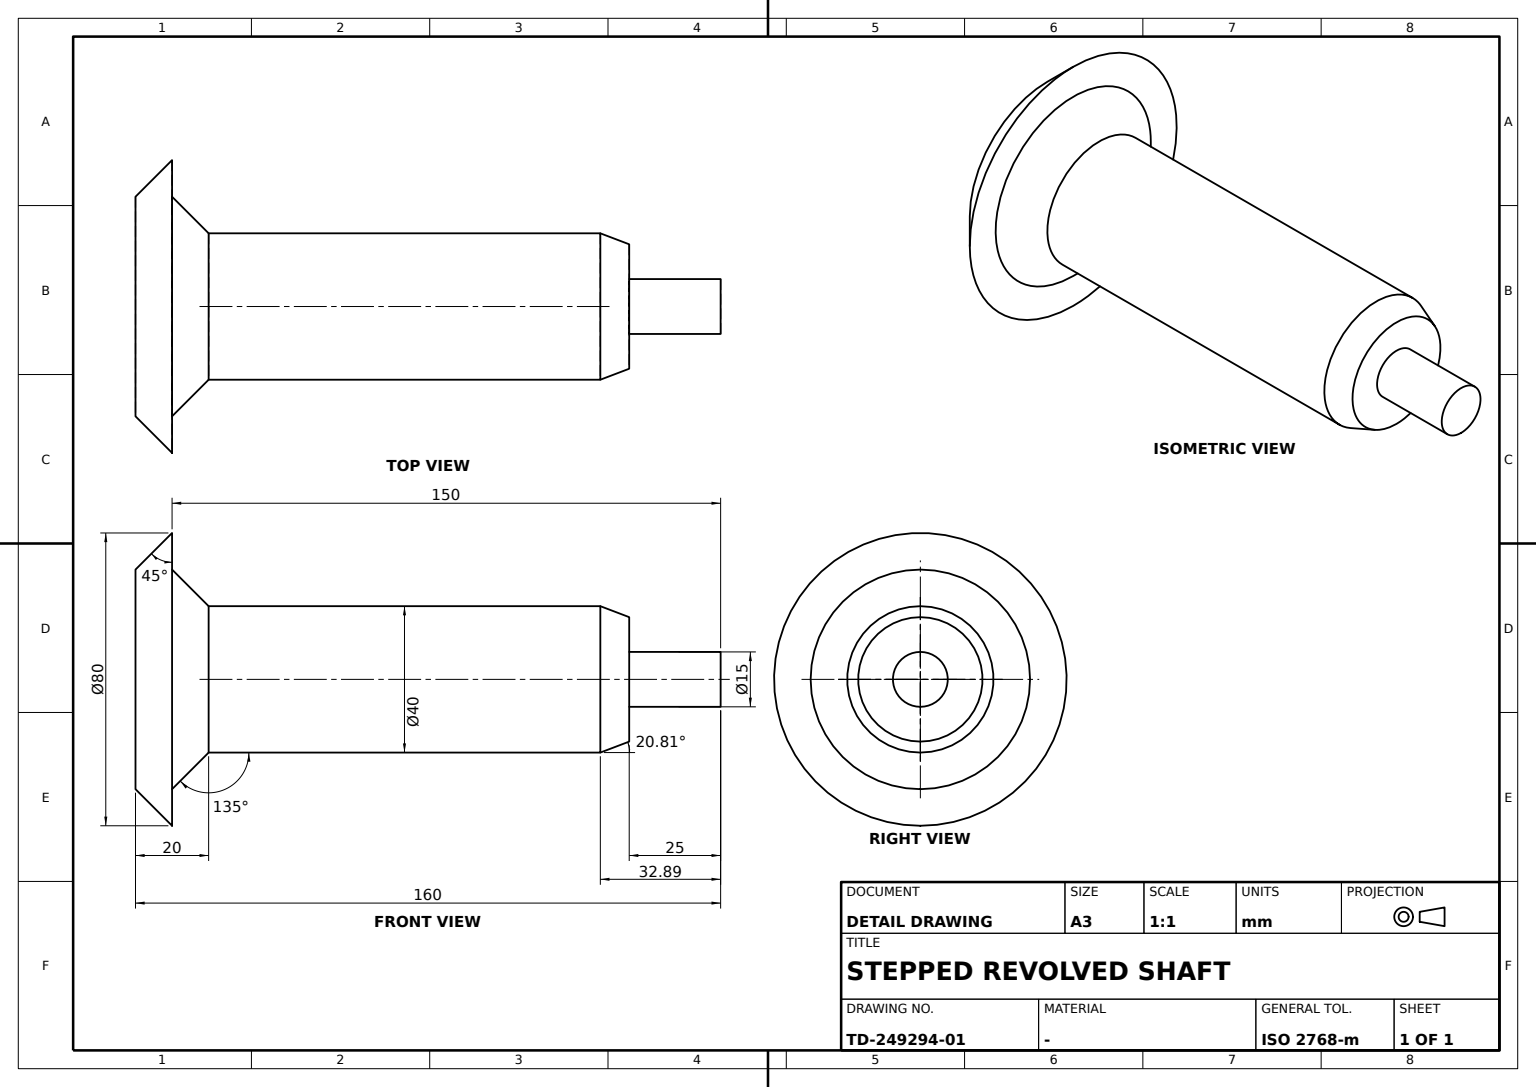
ISO-10303-21;
HEADER;
FILE_DESCRIPTION((''),'2;1');
FILE_NAME('','',(''),(''),'','','');
FILE_SCHEMA(('AUTOMOTIVE_DESIGN'));
ENDSEC;
DATA;
#1=APPLICATION_CONTEXT('');
#2=PRODUCT_CONTEXT('',#1,'mechanical');
#3=PRODUCT('','','',(#2));
#4=PRODUCT_DEFINITION_FORMATION('','',#3);
#5=PRODUCT_DEFINITION_CONTEXT('',#1,'design');
#6=PRODUCT_DEFINITION('','',#4,#5);
#7=PRODUCT_DEFINITION_SHAPE('','',#6);
#8=(LENGTH_UNIT()NAMED_UNIT(*)SI_UNIT(.MILLI.,.METRE.));
#9=(NAMED_UNIT(*)PLANE_ANGLE_UNIT()SI_UNIT($,.RADIAN.));
#10=(NAMED_UNIT(*)SI_UNIT($,.STERADIAN.)SOLID_ANGLE_UNIT());
#11=UNCERTAINTY_MEASURE_WITH_UNIT(LENGTH_MEASURE(0.005),#8,'distance_accuracy_value','');
#12=(GEOMETRIC_REPRESENTATION_CONTEXT(3)GLOBAL_UNCERTAINTY_ASSIGNED_CONTEXT((#11))GLOBAL_UNIT_ASSIGNED_CONTEXT((#8,#9,#10))REPRESENTATION_CONTEXT('',''));
#13=CARTESIAN_POINT('',(0.,-150.,-40.));
#14=VERTEX_POINT('',#13);
#15=CARTESIAN_POINT('',(0.,-150.,0.));
#16=DIRECTION('',(0.,-1.,0.));
#17=DIRECTION('',(0.,0.,-1.));
#18=AXIS2_PLACEMENT_3D('',#15,#16,#17);
#19=CIRCLE('',#18,40.);
#20=EDGE_CURVE('',#14,#14,#19,.T.);
#21=ORIENTED_EDGE('',*,*,#20,.F.);
#22=EDGE_LOOP('',(#21));
#23=FACE_BOUND('',#22,.T.);
#24=CARTESIAN_POINT('',(0.,-150.,-30.));
#25=VERTEX_POINT('',#24);
#26=CIRCLE('',#18,30.);
#27=EDGE_CURVE('',#25,#25,#26,.T.);
#28=ORIENTED_EDGE('',*,*,#27,.T.);
#29=EDGE_LOOP('',(#28));
#30=FACE_BOUND('',#29,.T.);
#31=CARTESIAN_POINT('',(0.,-150.,20.));
#32=DIRECTION('',(1.,0.,0.));
#33=AXIS2_PLACEMENT_3D('',#31,#16,#32);
#34=PLANE('',#33);
#35=ADVANCED_FACE('',(#23,#30),#34,.F.);
#36=CARTESIAN_POINT('',(0.,-25.,-7.5));
#37=VERTEX_POINT('',#36);
#38=CARTESIAN_POINT('',(0.,-25.,0.));
#39=AXIS2_PLACEMENT_3D('',#38,#16,#17);
#40=CIRCLE('',#39,7.5);
#41=EDGE_CURVE('',#37,#37,#40,.T.);
#42=ORIENTED_EDGE('',*,*,#41,.T.);
#43=EDGE_LOOP('',(#42));
#44=FACE_BOUND('',#43,.T.);
#45=CARTESIAN_POINT('',(0.,-25.,-17.));
#46=VERTEX_POINT('',#45);
#47=CIRCLE('',#39,17.);
#48=EDGE_CURVE('',#46,#46,#47,.T.);
#49=ORIENTED_EDGE('',*,*,#48,.F.);
#50=EDGE_LOOP('',(#49));
#51=FACE_BOUND('',#50,.T.);
#52=CARTESIAN_POINT('',(0.,-25.,7.5));
#53=AXIS2_PLACEMENT_3D('',#52,#16,#32);
#54=PLANE('',#53);
#55=ADVANCED_FACE('',(#44,#51),#54,.F.);
#56=CARTESIAN_POINT('',(0.,-140.,-20.));
#57=VERTEX_POINT('',#56);
#58=CARTESIAN_POINT('',(0.,-140.,0.));
#59=AXIS2_PLACEMENT_3D('',#58,#16,#17);
#60=CIRCLE('',#59,20.);
#61=EDGE_CURVE('',#57,#57,#60,.T.);
#62=ORIENTED_EDGE('',*,*,#61,.F.);
#63=EDGE_LOOP('',(#62));
#64=FACE_BOUND('',#63,.T.);
#65=CARTESIAN_POINT('',(0.,-32.894737,-20.));
#66=VERTEX_POINT('',#65);
#67=CARTESIAN_POINT('',(0.,-32.894737,0.));
#68=AXIS2_PLACEMENT_3D('',#67,#16,#17);
#69=CIRCLE('',#68,20.);
#70=EDGE_CURVE('',#66,#66,#69,.T.);
#71=ORIENTED_EDGE('',*,*,#70,.T.);
#72=EDGE_LOOP('',(#71));
#73=FACE_BOUND('',#72,.T.);
#74=CARTESIAN_POINT('',(0.,-80.,0.));
#75=AXIS2_PLACEMENT_3D('',#74,#16,#32);
#76=CYLINDRICAL_SURFACE('',#75,20.);
#77=ADVANCED_FACE('',(#64,#73),#76,.T.);
#78=ORIENTED_EDGE('',*,*,#61,.T.);
#79=EDGE_LOOP('',(#78));
#80=FACE_BOUND('',#79,.T.);
#81=ORIENTED_EDGE('',*,*,#27,.F.);
#82=EDGE_LOOP('',(#81));
#83=FACE_BOUND('',#82,.T.);
#84=CARTESIAN_POINT('',(0.,-120.,0.));
#85=DIRECTION('',(0.448263378,0.,-0.893901529));
#86=AXIS2_PLACEMENT_3D('',#84,#16,#85);
#87=CONICAL_SURFACE('',#86,0.,0.785398163);
#88=ADVANCED_FACE('',(#80,#83),#87,.T.);
#89=ORIENTED_EDGE('',*,*,#48,.T.);
#90=EDGE_LOOP('',(#89));
#91=FACE_BOUND('',#90,.T.);
#92=ORIENTED_EDGE('',*,*,#70,.F.);
#93=EDGE_LOOP('',(#92));
#94=FACE_BOUND('',#93,.T.);
#95=AXIS2_PLACEMENT_3D('',#38,#16,#32);
#96=CONICAL_SURFACE('',#95,17.,0.36314701);
#97=ADVANCED_FACE('',(#91,#94),#96,.T.);
#98=ORIENTED_EDGE('',*,*,#41,.F.);
#99=EDGE_LOOP('',(#98));
#100=FACE_BOUND('',#99,.T.);
#101=CARTESIAN_POINT('',(0.,0.,-7.5));
#102=VERTEX_POINT('',#101);
#103=CARTESIAN_POINT('',(0.,0.,0.));
#104=AXIS2_PLACEMENT_3D('',#103,#16,#17);
#105=CIRCLE('',#104,7.5);
#106=EDGE_CURVE('',#102,#102,#105,.T.);
#107=ORIENTED_EDGE('',*,*,#106,.T.);
#108=EDGE_LOOP('',(#107));
#109=FACE_BOUND('',#108,.T.);
#110=CYLINDRICAL_SURFACE('',#75,7.5);
#111=ADVANCED_FACE('',(#100,#109),#110,.T.);
#112=CARTESIAN_POINT('',(0.,-160.,-30.));
#113=VERTEX_POINT('',#112);
#114=CARTESIAN_POINT('',(0.,-160.,0.));
#115=AXIS2_PLACEMENT_3D('',#114,#16,#17);
#116=CIRCLE('',#115,30.);
#117=EDGE_CURVE('',#113,#113,#116,.T.);
#118=ORIENTED_EDGE('',*,*,#117,.T.);
#119=EDGE_LOOP('',(#118));
#120=FACE_BOUND('',#119,.T.);
#121=CARTESIAN_POINT('',(0.,-160.,40.));
#122=AXIS2_PLACEMENT_3D('',#121,#16,#32);
#123=PLANE('',#122);
#124=ADVANCED_FACE('',(#120),#123,.T.);
#125=ORIENTED_EDGE('',*,*,#106,.F.);
#126=EDGE_LOOP('',(#125));
#127=FACE_BOUND('',#126,.T.);
#128=AXIS2_PLACEMENT_3D('',#103,#16,#32);
#129=PLANE('',#128);
#130=ADVANCED_FACE('',(#127),#129,.F.);
#131=ORIENTED_EDGE('',*,*,#117,.F.);
#132=EDGE_LOOP('',(#131));
#133=FACE_BOUND('',#132,.T.);
#134=ORIENTED_EDGE('',*,*,#20,.T.);
#135=EDGE_LOOP('',(#134));
#136=FACE_BOUND('',#135,.T.);
#137=CARTESIAN_POINT('',(0.,-190.,0.));
#138=DIRECTION('',(0.,1.,0.));
#139=DIRECTION('',(0.479425539,0.,-0.877582562));
#140=AXIS2_PLACEMENT_3D('',#137,#138,#139);
#141=CONICAL_SURFACE('',#140,0.,0.785398163);
#142=ADVANCED_FACE('',(#133,#136),#141,.T.);
#143=CLOSED_SHELL('',(#35,#55,#77,#88,#97,#111,#124,#130,#142));
#144=MANIFOLD_SOLID_BREP('',#143);
#145=ADVANCED_BREP_SHAPE_REPRESENTATION('',(#144),#12);
#146=SHAPE_DEFINITION_REPRESENTATION(#7,#145);
ENDSEC;
END-ISO-10303-21;
